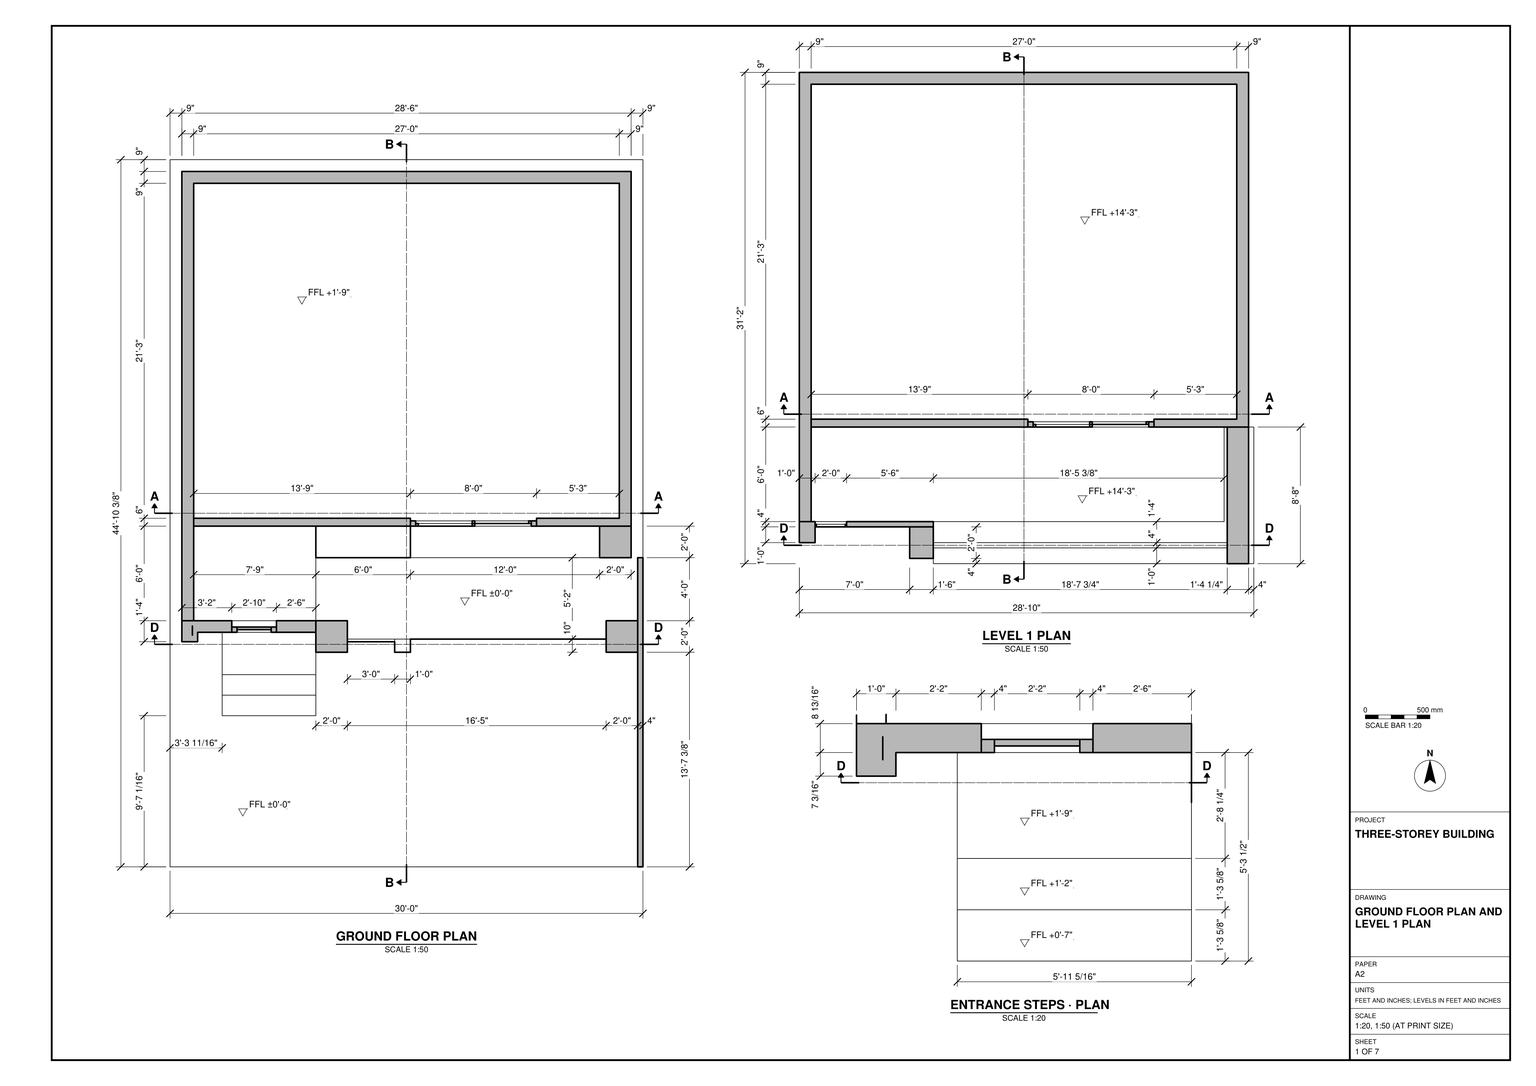
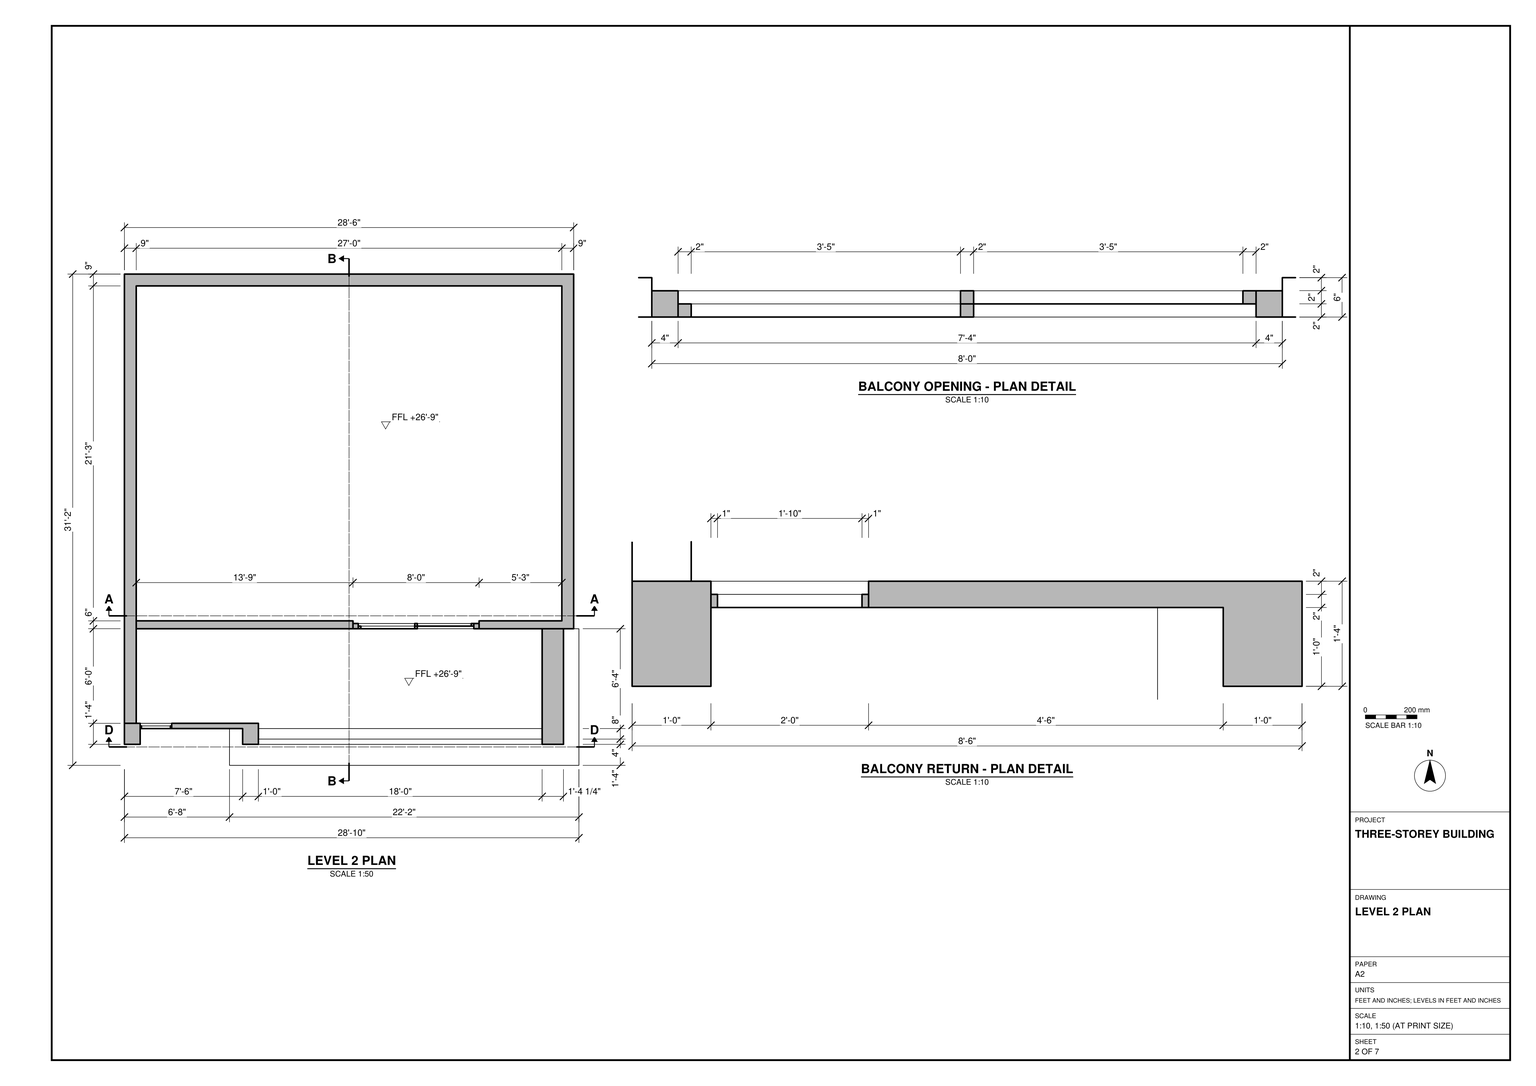
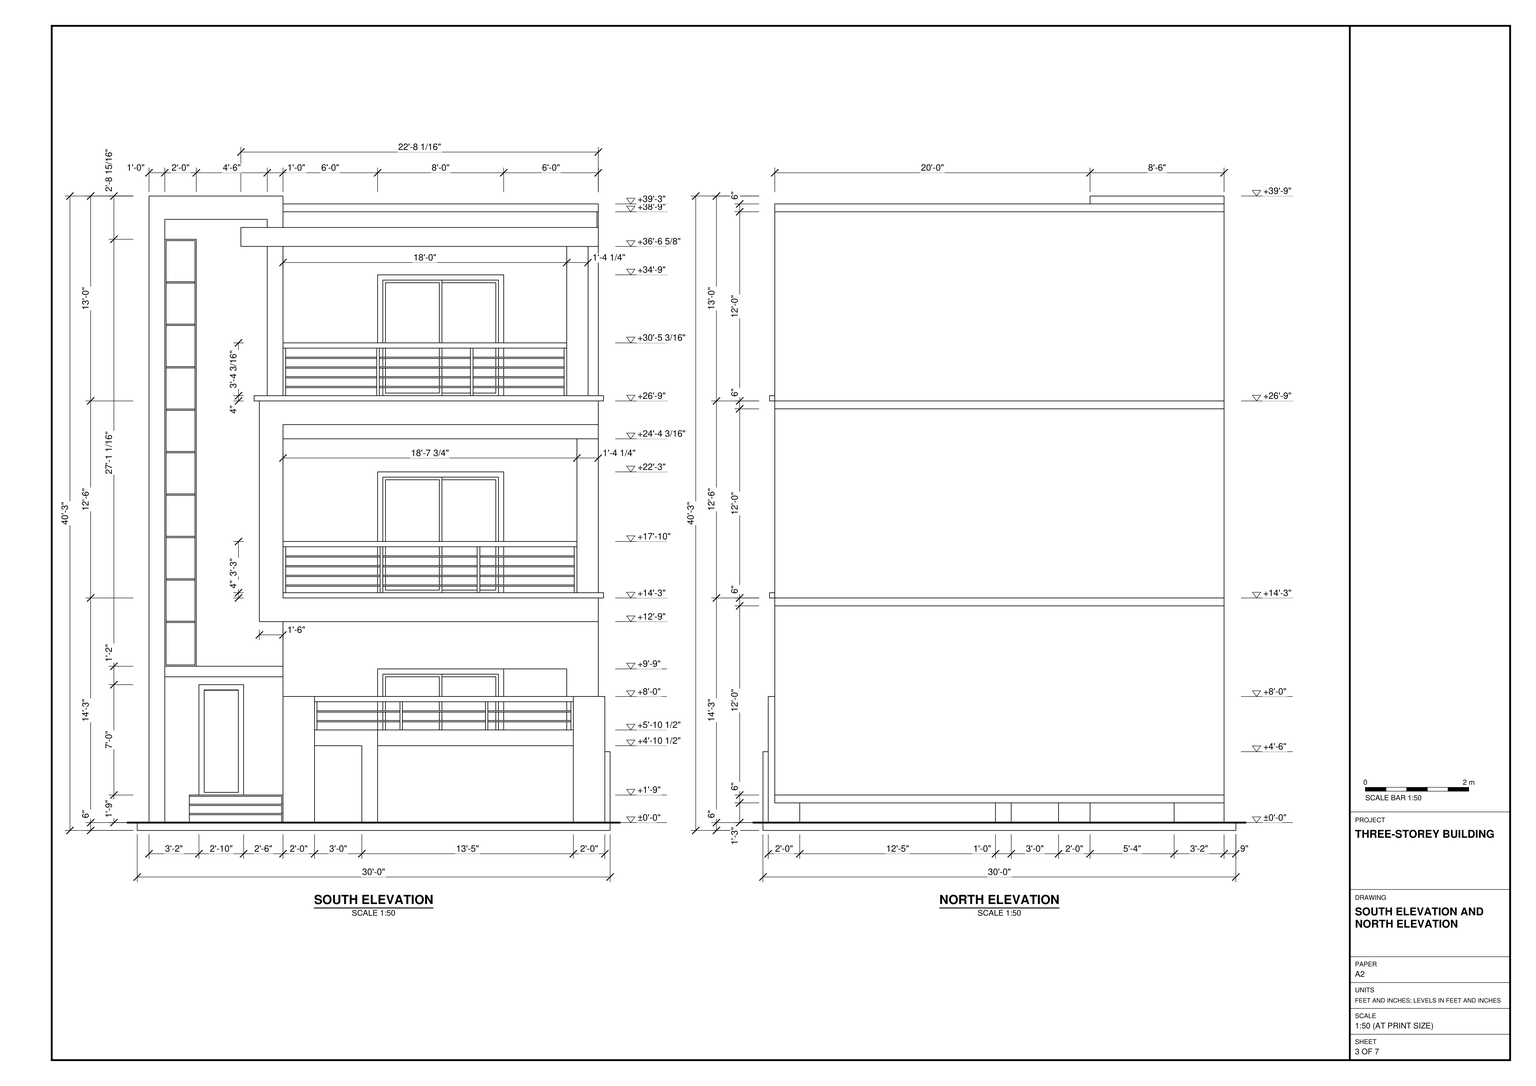
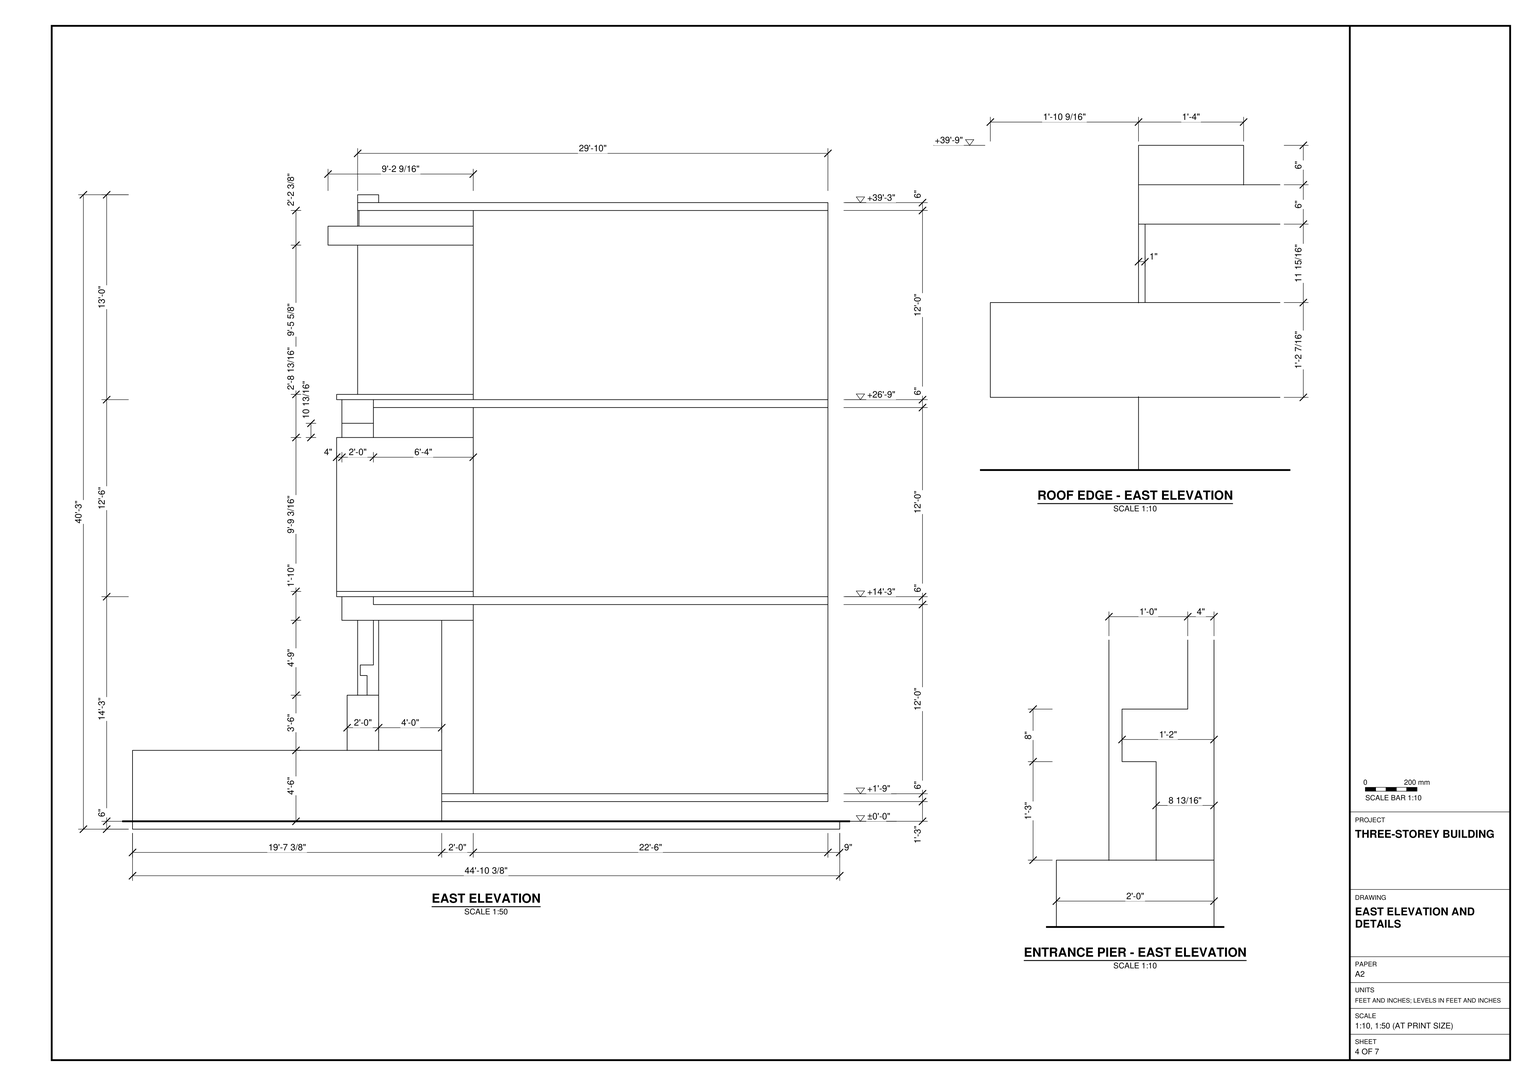
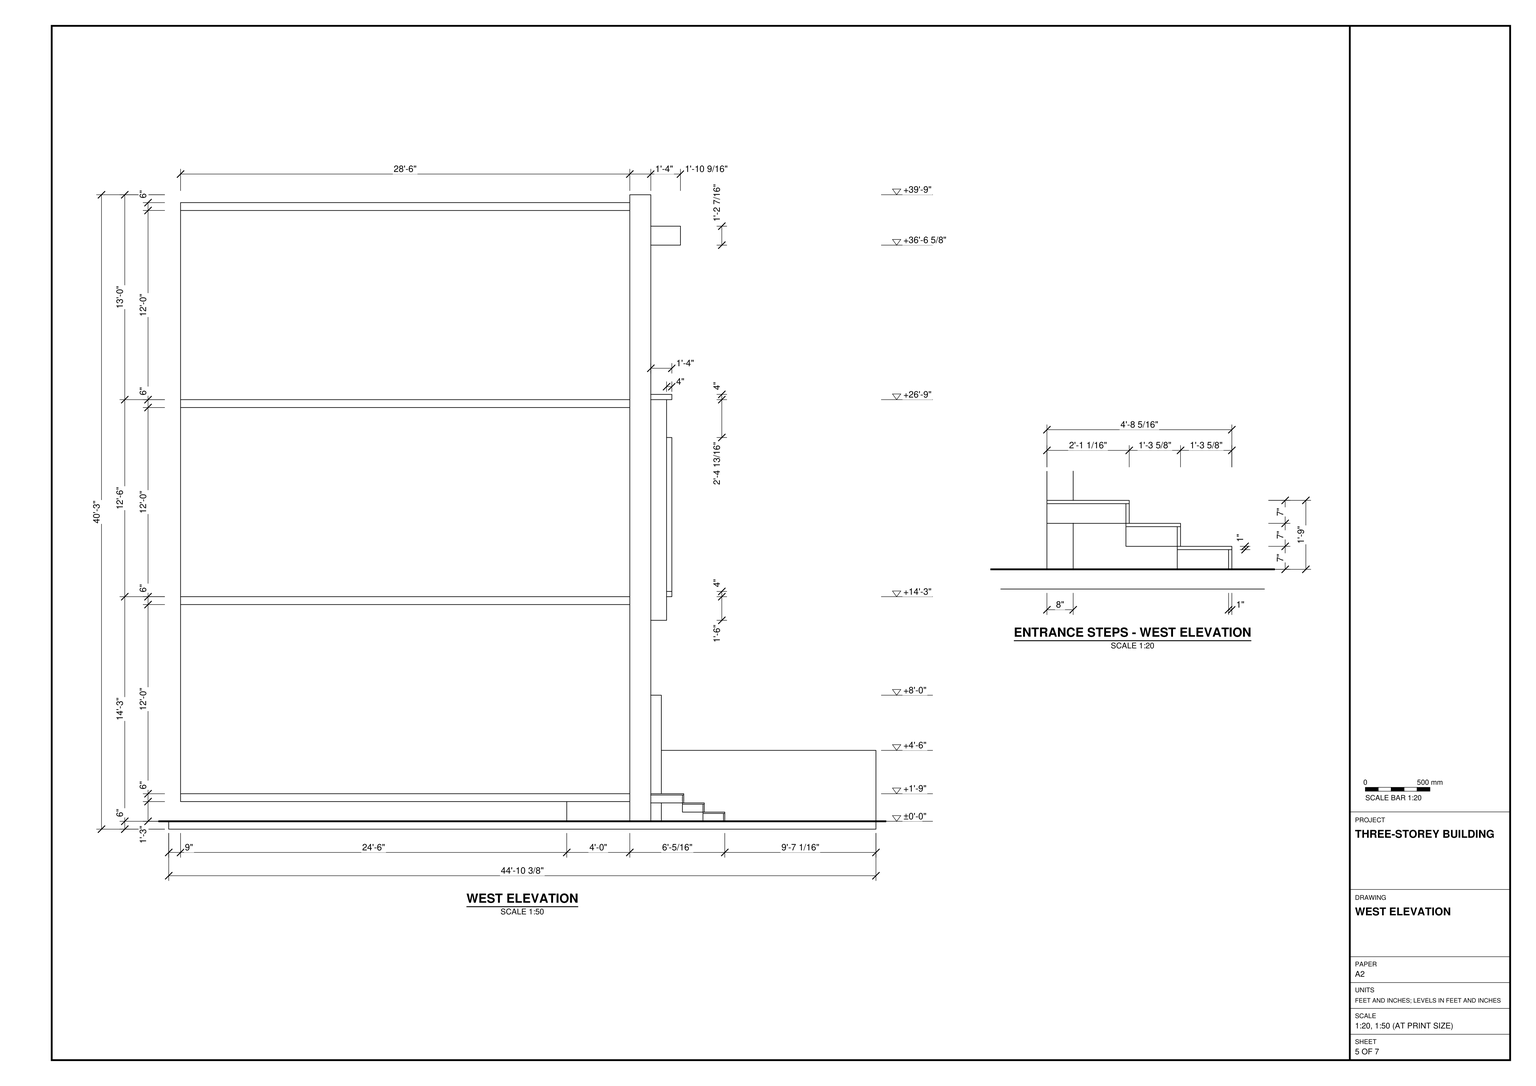
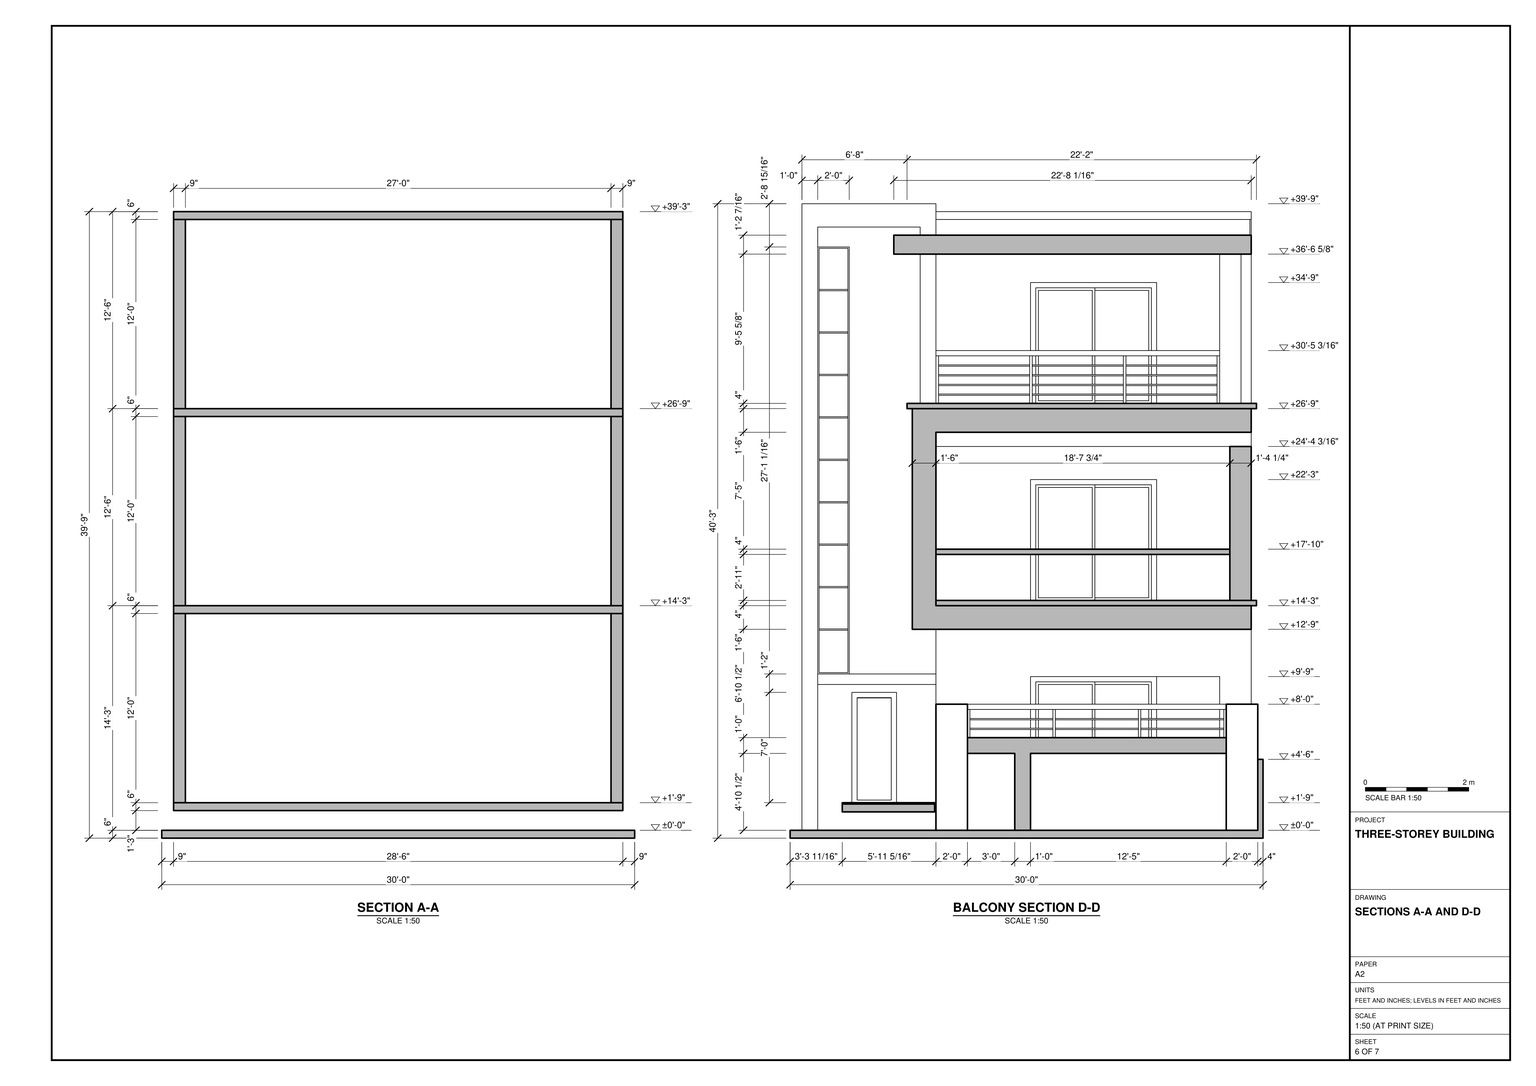
Build the three-storey building shown in task_files/diagram_01.pdf in SketchUp. Work in feet and inches. Include the base and front approach in the overall dimensions of 30'-0" wide, 44'-10 3/8" deep and 40'-3" high. Use ±0'-0" as the ground datum, with Level 1 at +14'-3" and Level 2 at +26'-9". The enclosed ground floor is raised above the approach to +1'-9".

Lay out the rectangular enclosed space on each floor with 9" side and rear walls and a 6" wall facing the front porch or balcony. Model the floor slabs, the entrance steps and landing on the left of the south elevation, and the screened porch beside them. Align the paired framed openings vertically behind the porch and balconies. Follow the separate upper-floor plans for the balcony slab edges, supports and short wall returns rather than copying one balcony unchanged. Include the horizontal railings, the tall narrow panel strip above the entrance, and the projecting band at the flat roof. Keep the rear elevation plain as drawn.

Keep walls, slabs and roof separate as groups or components, and do the same for each furniture or joinery piece shown. Use components for repeated parts. Any decor or loose items shown may use suitable library components. Save one SketchUp model as output_files/three_storey_building_with_stacked_front_balconies.skp.

# SketchUp Ruby script. Lengths in inches.
U = 1.inch
M = Sketchup.active_model
def pt(a) = Geom::Point3d.new(a.map { |v| v * U })
def face(e, loops, mat)
  f = e.add_face(loops[0].map { |a| pt(a) })
  loops[1..].each { |l| e.add_face(l.map { |a| pt(a) }).erase! }
  f.material = f.back_material = mat if mat
  f
end
# faces: each face lists its corners as indices into pts; further lists are holes
def faces(e, pts, list, mat = nil) = list.each { |f| face(e, (f[0].is_a?(Array) ? f : [f]).map { |l| l.map { |i| pts[i] } }, mat) }
# xy, xz, yz: faces in a plane at the given z, y or x. An outline is a flat list of corners, or four numbers for a rectangle; further outlines are holes
def ring(l) = l.size == 4 ? [[l[0], l[1]], [l[2], l[1]], [l[2], l[3]], [l[0], l[3]]] : l.each_slice(2).to_a
def flat(e, list, mat, &to3) = list.each { |f| face(e, (f[0].is_a?(Array) ? f : [f]).map { |l| ring(l).map { |u, v| to3.(u, v) } }, mat) }
def xy(e, z, list, mat = nil) = flat(e, list, mat) { |x, y| [x, y, z] }
def xz(e, y, list, mat = nil) = flat(e, list, mat) { |x, z| [x, y, z] }
def yz(e, x, list, mat = nil) = flat(e, list, mat) { |y, z| [x, y, z] }
def lines(e, pts, list) = list.each { |a, b| e.add_line(pt(pts[a]), pt(pts[b])) }
# prism: a flat outline (further loops are holes) pulled along v
def prism(e, loops, v, mat = nil)
  f = face(e, loops, mat); d = Geom::Vector3d.new(v.map { |x| x * U })
  f.pushpull(f.normal.samedirection?(d) ? d.length : -d.length)
end
def box(e, o, s, mat = nil) = prism(e, [[o, [o[0] + s[0], o[1], o[2]], [o[0] + s[0], o[1] + s[1], o[2]], [o[0], o[1] + s[1], o[2]]]], [0, 0, s[2]], mat)
def at(x, y, z, deg = 0) = Geom::Transformation.translation(pt([x, y, z])) * Geom::Transformation.rotation(ORIGIN, Z_AXIS, deg.degrees)
def axes(o, x, y, z) = Geom::Transformation.new([*x, 0, *y, 0, *z, 0, *pt(o).to_a, 1])
def part(name) = M.definitions.add(name)
# library, detail: a bought-in or finely detailed component or shape, given as its bounding box
def library(name, o, s) = part(name).tap { |d| box(d.entities, o, s) }
def detail(e, o, s) = box(e.add_group.entities, o, s)
def put(e, d, t, mat = nil) = e.add_instance(d, t).tap { |i| i.material = mat if mat }
def group(e, t, mat = nil) = e.add_group.tap { |g| g.transformation = t; g.material = mat if mat }.entities
root = M.entities
M.materials.add("[Carpet Berber Pattern Gray]").color = [165, 165, 165]
M.materials.add("[Color K02]").color = [255, 153, 255]
M.materials.add("[Color M05]").color = [114, 114, 114]
M.materials.add("[Color M06]").color = [86, 86, 86]
M.materials.add("[Color M07]").color = [58, 58, 58]
M.materials.add("[Concrete Tile]").color = [163, 163, 163]
M.materials.add("[Fabric Linen]").color = [161, 161, 136]
M.materials.add("[Roofing Slate Tan]").color = [200, 175, 128]
M.materials.add("[Sketchy Siding Scale]").color = [244, 244, 244]
M.materials.add("[Sketchy Stone Ashlar]").color = [168, 168, 168]
M.materials.add("[Slate Light Tile]").color = [54, 54, 54]
M.materials.add("[Translucent Glass Gray]").color = [128, 128, 128]
M.materials["[Translucent Glass Gray]"].alpha = 0.86
M.materials.add("[Translucent Glass Gray]1").color = [33, 33, 33]
M.materials["[Translucent Glass Gray]1"].alpha = 0.5
M.materials.add("[Wood Floor Light]").color = [197, 155, 82]
c1 = part("Group\#10")
g1 = group(c1.entities,at(4,0,4))
xy(g1,0,[[0,0,45,2]])
xy(g1,2,[[2,0,43,2]])
xy(g1,86,[[2,0,43,2]])
xy(g1,88,[[0,0,45,2]])
xz(g1,0,[[[0,0,45,88],[2,2,43,86]]])
xz(g1,0,[[2,2,43,86]],"[Translucent Glass Gray]")
xz(g1,2,[[[0,0,45,88],[2,2,43,86]]])
yz(g1,0,[[0,0,2,88]])
yz(g1,2,[[0,2,2,86]])
yz(g1,43,[[0,2,2,86]])
yz(g1,45,[[0,0,2,88]])
g2 = group(c1.entities,at(47,2,4))
xy(g2,0,[[0,0,45,2]])
xy(g2,2,[[2,0,43,2]])
xy(g2,86,[[2,0,43,2]])
xy(g2,88,[[0,0,45,2]])
xz(g2,0,[[[0,0,45,88],[2,2,43,86]]])
xz(g2,0,[[2,2,43,86]],"[Translucent Glass Gray]")
xz(g2,2,[[[0,0,45,88],[2,2,43,86]]])
yz(g2,0,[[0,0,2,88]])
yz(g2,2,[[0,2,2,86]])
yz(g2,43,[[0,2,2,86]])
yz(g2,45,[[0,0,2,88]])
g3 = group(c1.entities,at(0,0,0))
prism(g3,[[[0,4,96],[96,4,96],[96,4,0],[0,4,0]],[[4,4,4],[92,4,4],[92,4,92],[4,4,92]]],[0,-4,0])
c2 = part("Group\#20")
box(c2.entities,[0,0,0],[24,24,96])
g4 = group(root,at(0,178.375,0))
xy(g4,-6,[[0,-178.375,360,360]])
xy(g4,0,[[0,-178.375,356,-178.375,356,57,360,57,360,360,0,360]],"[Sketchy Stone Ashlar]")
xy(g4,54,[[356,-178.375,360,57]],"[Color M05]")
xz(g4,-178.375,[[0,-6,360,-6,360,54,356,54,356,0,0,0]],"[Color M05]")
xz(g4,57,[[356,0,360,54]])
xz(g4,360,[[0,-6,360,0]])
yz(g4,0,[[-178.375,-6,360,0]])
yz(g4,356,[[-178.375,0,57,54]],"[Color M05]")
yz(g4,360,[[-178.375,-6,360,-6,360,0,57,0,57,54,-178.375,54]],"[Color M05]")
g5 = group(root,at(9,106.75,15))
prism(g5,[[[0,422.625,0],[342,422.625,0],[342,128.625,0],[102,128.625,0],[102,80.625,0],[0,80.625,0]]],[0,0,6])
p = [[333,413.625,6],[9,413.625,6]]
lines(g5,p,[[0,1]])
g6 = group(root,at(9,171.375,21),"[Sketchy Siding Scale]")
xy(g6,-21,[[0,0,0,12,8,12,8,5,12,5,12,0],[8,5,8,12,0,12,0,16,38,16,38,7.1875,12,7.1875,12,5],[38,7.1875,102,16]])
xy(g6,0,[[38,7.1875,72,16]])
xy(g6,84,[[38,7.1875,72,16]])
xy(g6,90,[[8,2,12,5]])
xy(g6,90,[[12,2,102,7.1875]],"[Color M06]")
xy(g6,98,[[8,2,12,12]])
xy(g6,98,[[12,2,102,2,102,12,36,12,36,16,12,16]],"[Color M06]")
xy(g6,300,[[90,0,102,12]])
xy(g6,423.0625,[[12,12,36,16]])
xy(g6,438.25,[[12,0,90,12]],"[Color M06]")
xy(g6,456,[[0,0,102,16]],"[Color M06]")
xz(g6,0,[[0,-21,12,-21,12,438.25,90,438.25,90,300,102,300,102,456,0,456]],"[Color M06]")
xz(g6,2,[[8,90,12,98]])
xz(g6,2,[[12,90,102,98]],"[Color M06]")
xz(g6,7.1875,[[[12,-21,102,90],[38,0,72,84]]])
xz(g6,12,[[36,98,102,98,102,300,90,300,90,438.25,12,438.25,12,423.0625,36,423.0625]],"[Concrete Tile]")
xz(g6,16,[[[0,-21,0,456,102,456,102,-21,38,-21,38,0,72,0,72,84,38,84,38,-21],[12,98,36,423.0625]]])
yz(g6,0,[[0,-21,16,456]],"[Color M06]")
yz(g6,8,[[5,-21,12,90],[2,90,12,98]])
yz(g6,12,[[0,-21,7.1875,-21,7.1875,90,2,90,2,98,16,98,16,423.0625,12,423.0625,12,438.25,0,438.25]])
yz(g6,36,[[12,98,16,423.0625]])
yz(g6,38,[[7.1875,0,16,84]])
yz(g6,72,[[7.1875,0,16,84]])
yz(g6,90,[[0,300,12,438.25]],"[Color M06]")
yz(g6,102,[[7.1875,-21,16,-21,16,456,0,456,0,300,12,300,12,98,2,98,2,90,7.1875,90]],"[Color M06]")
g7 = group(root,at(93,159.375,153),"[Color M07]")
xy(g7,0,[[0,0,0,24,18,24,18,100,258,100,258,0]])
xy(g7,12,[[18,24,258,100]])
xy(g7,18,[[18,0,258,24]])
xy(g7,150,[[18,0,258,24]])
xy(g7,168,[[0,0,258,24]])
xz(g7,0,[[0,0,258,0,258,18,18,18,18,150,258,150,258,168,0,168]])
xz(g7,24,[[0,0,0,168,258,168,258,150,18,150,18,18,258,18,258,12,18,12,18,0]])
xz(g7,100,[[18,0,258,12]])
yz(g7,0,[[0,0,24,168]])
yz(g7,18,[[24,0,100,12],[0,18,24,150]])
yz(g7,258,[[0,0,100,0,100,12,24,12,24,18,0,18],[0,150,24,168]])
g8 = group(root,at(9,187.375,21))
xy(g8,0,[[0,0,0,342,342,342,342,72,270,72,270,78,333,78,333,333,9,333,9,0],[9,72,174,78]])
xy(g8,96,[[174,72,270,78]])
xy(g8,144,[[[0,0,9,0,9,72,342,72,342,342,0,342],[9,78,333,333]]])
xz(g8,0,[[0,0,9,144]])
xz(g8,72,[[9,0,174,0,174,96,270,96,270,0,342,0,342,144,9,144]],"[Roofing Slate Tan]")
xz(g8,78,[[9,0,9,144,333,144,333,0,270,0,270,96,174,96,174,0]])
xz(g8,333,[[9,0,333,144]])
xz(g8,342,[[0,0,342,144]])
yz(g8,0,[[0,0,342,144]])
yz(g8,9,[[0,0,72,144],[72,0,78,144],[78,0,333,144]])
yz(g8,174,[[72,0,78,96]])
yz(g8,270,[[72,0,78,96]])
yz(g8,333,[[78,0,333,144]])
yz(g8,342,[[72,0,342,144]])
put(root,c1,at(183,259.375,21),"[Slate Light Tile]")
g9 = group(root,at(9,187.375,171))
xy(g9,0,[[0,0,0,342,342,342,342,72,270,72,270,78,333,78,333,333,9,333,9,0],[9,72,174,78]])
xy(g9,96,[[174,72,270,78]])
xy(g9,144,[[[0,0,9,0,9,72,342,72,342,342,0,342],[9,78,333,333]]])
xz(g9,0,[[0,0,9,144]])
xz(g9,72,[[9,0,174,0,174,96,270,96,270,0,342,0,342,144,9,144]],"[Wood Floor Light]")
xz(g9,78,[[9,0,9,144,333,144,333,0,270,0,270,96,174,96,174,0]])
xz(g9,333,[[9,0,333,144]])
xz(g9,342,[[0,0,342,144]])
yz(g9,0,[[0,0,342,144]])
yz(g9,9,[[0,0,72,144],[72,0,78,144],[78,0,333,144]])
yz(g9,174,[[72,0,78,96]])
yz(g9,270,[[72,0,78,96]])
yz(g9,333,[[78,0,333,144]])
yz(g9,342,[[72,0,342,144]])
g10 = group(root,at(9,183.375,315))
prism(g10,[[[0,346,0],[342,346,0],[342,0,0],[102,0,0],[102,4,0],[0,4,0]]],[0,0,6])
put(root,c1,at(183,259.375,171),"[Slate Light Tile]")
g11 = group(root,at(9,187.375,321))
xy(g11,0,[[0,0,0,342,342,342,342,72,270,72,270,78,333,78,333,333,9,333,9,0],[9,72,174,78]])
xy(g11,96,[[174,72,270,78]])
xy(g11,144,[[[0,0,9,0,9,72,342,72,342,342,0,342],[9,78,333,333]]])
xz(g11,0,[[0,0,9,144]])
xz(g11,72,[[9,0,174,0,174,96,270,96,270,0,342,0,342,144,9,144]],"[Fabric Linen]")
xz(g11,78,[[9,0,9,144,333,144,333,0,270,0,270,96,174,96,174,0]])
xz(g11,333,[[9,0,333,144]])
xz(g11,342,[[0,0,342,144]])
yz(g11,0,[[0,0,342,144]])
yz(g11,9,[[0,0,72,144],[72,0,78,144],[78,0,333,144]])
yz(g11,174,[[72,0,78,96]])
yz(g11,270,[[72,0,78,96]])
yz(g11,333,[[78,0,333,144]])
yz(g11,342,[[72,0,342,144]])
g12 = group(root,at(9,183.375,465),"[Color M06]")
prism(g12,[[[0,346,0],[342,346,0],[342,-12,0],[102,-12,0],[102,4,0],[0,4,0]]],[0,0,6])
put(root,c1,at(183,259.375,321),"[Slate Light Tile]")
g13 = group(root,at(111,235.375,21),"[Carpet Berber Pattern Gray]")
prism(g13,[[[216,24,96],[72,24,96],[72,24,0],[0,24,0],[0,24,132],[240,24,132],[240,24,0],[216,24,0]]],[0,-24,0])
g14 = group(root,at(9,183.375,165))
prism(g14,[[[0,346,0],[342,346,0],[342,0,0],[102,0,0],[102,4,0],[0,4,0]]],[0,0,6])
g15 = group(root,at(111,155.375,171),"[Color M07]")
prism(g15,[[[244,104,0],[244,0,0],[0,0,0],[0,32,0],[221.375,32,0],[221.375,104,0]]],[0,0,4])
g16 = group(root,at(111,183.375,292.1875),"[Sketchy Siding Scale]")
xy(g16,0,[[0,0,240,76]],"[Wood Floor Light]")
xy(g16,22.8125,[[0,0,240,76]])
xz(g16,0,[[0,0,240,22.8125]])
xz(g16,76,[[0,0,240,22.8125]])
yz(g16,0,[[0,0,76,22.8125]])
yz(g16,240,[[0,0,76,22.8125]])
g17 = group(root,at(334.75,155.375,175),"[Color M06]")
box(g17,[0,0,0],[16.25,104,117.1875])
g18 = group(root,at(93,159.375,321),"[Color M07]")
prism(g18,[[[-4,24,0],[6,24,0],[6,12,0],[18,12,0],[18,24,0],[234,24,0],[234,100,0],[262,100,0],[262,-4,0],[-4,-4,0]]],[0,0,4])
g19 = group(root,at(327,155.375,325),"[Color M06]")
box(g19,[0,16,0],[16.25,88,117.1875])
g20 = group(root,at(111,167.375,173),"[Slate Light Tile]")
xy(g20,0,[[0,0,2.07,2],[73.89,0,75.96,2],[147.79,0,149.86,2],[221.68,0,223.75,2]])
xy(g20,6.9,[[0,1,73.89,2],[73.89,1,147.79,2],[147.79,1,221.68,2],[221.68,1,223.75,2]])
xy(g20,7.9,[[0,1,73.89,2],[73.89,1,147.79,2],[147.79,1,221.68,2],[221.68,1,223.75,2]])
xy(g20,14.3,[[0,1,73.89,2],[73.89,1,147.79,2],[147.79,1,221.68,2],[221.68,1,223.75,2]])
xy(g20,15.3,[[0,1,73.89,2],[73.89,1,147.79,2],[147.79,1,221.68,2],[221.68,1,223.75,2]])
xy(g20,21.7,[[0,1,73.89,2],[73.89,1,147.79,2],[147.79,1,221.68,2],[221.68,1,223.75,2]])
xy(g20,22.7,[[0,1,73.89,2],[73.89,1,147.79,2],[147.79,1,221.68,2],[221.68,1,223.75,2]])
xy(g20,29.1,[[0,1,73.89,2],[73.89,1,147.79,2],[147.79,1,221.68,2],[221.68,1,223.75,2]])
xy(g20,30.1,[[0,1,73.89,2],[73.89,1,147.79,2],[147.79,1,221.68,2],[221.68,1,223.75,2]])
xy(g20,37,[[2.07,0,2.07,2,0,2,0,4,223.75,4,223.75,2,221.68,2,221.68,0,149.86,0,149.86,2,147.79,2,147.79,0,75.96,0,75.96,2,73.89,2,73.89,0],[73.89,0,75.96,2],[147.79,0,149.86,2],[221.68,0,223.75,2]])
xy(g20,41,[[0,0,223.75,4]])
xz(g20,0,[[0,0,2.07,37],[73.89,0,75.96,37],[147.79,0,149.86,37],[221.68,0,223.75,37],[0,37,223.75,41]])
xz(g20,1,[[0,6.9,73.89,7.9],[73.89,6.9,147.79,7.9],[147.79,6.9,221.68,7.9],[221.68,6.9,223.75,7.9],[0,14.3,73.89,15.3],
  [73.89,14.3,147.79,15.3],[147.79,14.3,221.68,15.3],[221.68,14.3,223.75,15.3],[0,21.7,73.89,22.7],[73.89,21.7,147.79,22.7],
  [147.79,21.7,221.68,22.7],[221.68,21.7,223.75,22.7],[0,29.1,73.89,30.1],[73.89,29.1,147.79,30.1],[147.79,29.1,221.68,30.1],
  [221.68,29.1,223.75,30.1]])
xz(g20,2,[[0,0,2.07,6.9],[73.89,0,75.96,6.9],[147.79,0,149.86,6.9],[221.68,0,223.75,6.9],[0,6.9,2.07,7.9],
  [2.07,6.9,73.89,7.9],[73.89,6.9,75.96,7.9],[75.96,6.9,147.79,7.9],[147.79,6.9,149.86,7.9],[149.86,6.9,221.68,7.9],
  [221.68,6.9,223.75,7.9],[0,7.9,2.07,14.3],[73.89,7.9,75.96,14.3],[147.79,7.9,149.86,14.3],[221.68,7.9,223.75,14.3],
  [0,14.3,2.07,15.3],[2.07,14.3,73.89,15.3],[73.89,14.3,75.96,15.3],[75.96,14.3,147.79,15.3],[147.79,14.3,149.86,15.3],
  [149.86,14.3,221.68,15.3],[221.68,14.3,223.75,15.3],[0,15.3,2.07,21.7],[73.89,15.3,75.96,21.7],[147.79,15.3,149.86,21.7],
  [221.68,15.3,223.75,21.7],[0,21.7,2.07,22.7],[2.07,21.7,73.89,22.7],[73.89,21.7,75.96,22.7],[75.96,21.7,147.79,22.7],
  [147.79,21.7,149.86,22.7],[149.86,21.7,221.68,22.7],[221.68,21.7,223.75,22.7],[0,22.7,2.07,29.1],[73.89,22.7,75.96,29.1],
  [147.79,22.7,149.86,29.1],[221.68,22.7,223.75,29.1],[0,29.1,2.07,30.1],[2.07,29.1,73.89,30.1],[73.89,29.1,75.96,30.1],
  [75.96,29.1,147.79,30.1],[147.79,29.1,149.86,30.1],[149.86,29.1,221.68,30.1],[221.68,29.1,223.75,30.1],[0,30.1,2.07,37],
  [73.89,30.1,75.96,37],[147.79,30.1,149.86,37],[221.68,30.1,223.75,37]])
xz(g20,4,[[0,37,223.75,41]])
yz(g20,0,[[0,0,0,37,2,37,2,30.1,1,30.1,1,29.1,2,29.1,2,22.7,1,22.7,1,21.7,2,21.7,2,15.3,1,15.3,1,14.3,2,14.3,2,7.9,1,7.9,1,6.9,2,6.9,2,0],[1,6.9,2,7.9],[1,14.3,2,15.3],[1,21.7,2,22.7],[1,29.1,2,30.1],
  [0,37,4,41]])
yz(g20,2.07,[[0,0,2,37]])
yz(g20,73.89,[[0,0,0,37,2,37,2,30.1,1,30.1,1,29.1,2,29.1,2,22.7,1,22.7,1,21.7,2,21.7,2,15.3,1,15.3,1,14.3,2,14.3,2,7.9,1,7.9,1,6.9,2,6.9,2,0],[1,6.9,2,7.9],[1,14.3,2,15.3],[1,21.7,2,22.7],[1,29.1,2,30.1]])
yz(g20,75.96,[[0,0,2,37]])
yz(g20,147.79,[[0,0,0,37,2,37,2,30.1,1,30.1,1,29.1,2,29.1,2,22.7,1,22.7,1,21.7,2,21.7,2,15.3,1,15.3,1,14.3,2,14.3,2,7.9,1,7.9,1,6.9,2,6.9,2,0],[1,6.9,2,7.9],[1,14.3,2,15.3],[1,21.7,2,22.7],[1,29.1,2,30.1]])
yz(g20,149.86,[[0,0,2,37]])
yz(g20,221.68,[[0,0,0,37,2,37,2,30.1,1,30.1,1,29.1,2,29.1,2,22.7,1,22.7,1,21.7,2,21.7,2,15.3,1,15.3,1,14.3,2,14.3,2,7.9,1,7.9,1,6.9,2,6.9,2,0],[1,6.9,2,7.9],[1,14.3,2,15.3],[1,21.7,2,22.7],[1,29.1,2,30.1]])
yz(g20,223.75,[[0,0,2,0,2,6.9,1,6.9,1,7.9,2,7.9,2,14.3,1,14.3,1,15.3,2,15.3,2,21.7,1,21.7,1,22.7,2,22.7,2,29.1,1,29.1,1,30.1,2,30.1,2,37,0,37],[1,6.9,2,7.9],[1,14.3,2,15.3],[1,21.7,2,22.7],[1,29.1,2,30.1],
  [0,37,4,41]])
g21 = group(root,at(111,171.375,324.22),"[Slate Light Tile]")
xy(g21,0,[[0,0,2,2],[71.33,0,73.33,2],[142.67,0,144.67,2],[214,0,216,2]])
xy(g21,6.9,[[0,1,71.33,2],[71.33,1,142.67,2],[142.67,1,214,2],[214,1,216,2]])
xy(g21,7.9,[[0,1,71.33,2],[71.33,1,142.67,2],[142.67,1,214,2],[214,1,216,2]])
xy(g21,14.3,[[0,1,71.33,2],[71.33,1,142.67,2],[142.67,1,214,2],[214,1,216,2]])
xy(g21,15.3,[[0,1,71.33,2],[71.33,1,142.67,2],[142.67,1,214,2],[214,1,216,2]])
xy(g21,21.7,[[0,1,71.33,2],[71.33,1,142.67,2],[142.67,1,214,2],[214,1,216,2]])
xy(g21,22.7,[[0,1,71.33,2],[71.33,1,142.67,2],[142.67,1,214,2],[214,1,216,2]])
xy(g21,29.1,[[0,1,71.33,2],[71.33,1,142.67,2],[142.67,1,214,2],[214,1,216,2]])
xy(g21,30.1,[[0,1,71.33,2],[71.33,1,142.67,2],[142.67,1,214,2],[214,1,216,2]])
xy(g21,37,[[2,0,2,2,0,2,0,4,216,4,216,2,214,2,214,0,144.67,0,144.67,2,142.67,2,142.67,0,73.33,0,73.33,2,71.33,2,71.33,0],[71.33,0,73.33,2],[142.67,0,144.67,2],[214,0,216,2]])
xy(g21,41,[[0,0,216,4]])
xz(g21,0,[[0,0,2,37],[71.33,0,73.33,37],[142.67,0,144.67,37],[214,0,216,37],[0,37,216,41]])
xz(g21,1,[[0,6.9,71.33,7.9],[71.33,6.9,142.67,7.9],[142.67,6.9,214,7.9],[214,6.9,216,7.9],[0,14.3,71.33,15.3],
  [71.33,14.3,142.67,15.3],[142.67,14.3,214,15.3],[214,14.3,216,15.3],[0,21.7,71.33,22.7],[71.33,21.7,142.67,22.7],
  [142.67,21.7,214,22.7],[214,21.7,216,22.7],[0,29.1,71.33,30.1],[71.33,29.1,142.67,30.1],[142.67,29.1,214,30.1],
  [214,29.1,216,30.1]])
xz(g21,2,[[0,0,2,6.9],[71.33,0,73.33,6.9],[142.67,0,144.67,6.9],[214,0,216,6.9],[0,6.9,2,7.9],
  [2,6.9,71.33,7.9],[71.33,6.9,73.33,7.9],[73.33,6.9,142.67,7.9],[142.67,6.9,144.67,7.9],[144.67,6.9,214,7.9],
  [214,6.9,216,7.9],[0,7.9,2,14.3],[71.33,7.9,73.33,14.3],[142.67,7.9,144.67,14.3],[214,7.9,216,14.3],
  [0,14.3,2,15.3],[2,14.3,71.33,15.3],[71.33,14.3,73.33,15.3],[73.33,14.3,142.67,15.3],[142.67,14.3,144.67,15.3],
  [144.67,14.3,214,15.3],[214,14.3,216,15.3],[0,15.3,2,21.7],[71.33,15.3,73.33,21.7],[142.67,15.3,144.67,21.7],
  [214,15.3,216,21.7],[0,21.7,2,22.7],[2,21.7,71.33,22.7],[71.33,21.7,73.33,22.7],[73.33,21.7,142.67,22.7],
  [142.67,21.7,144.67,22.7],[144.67,21.7,214,22.7],[214,21.7,216,22.7],[0,22.7,2,29.1],[71.33,22.7,73.33,29.1],
  [142.67,22.7,144.67,29.1],[214,22.7,216,29.1],[0,29.1,2,30.1],[2,29.1,71.33,30.1],[71.33,29.1,73.33,30.1],
  [73.33,29.1,142.67,30.1],[142.67,29.1,144.67,30.1],[144.67,29.1,214,30.1],[214,29.1,216,30.1],[0,30.1,2,37],
  [71.33,30.1,73.33,37],[142.67,30.1,144.67,37],[214,30.1,216,37]])
xz(g21,4,[[0,37,216,41]])
yz(g21,0,[[0,0,0,37,2,37,2,30.1,1,30.1,1,29.1,2,29.1,2,22.7,1,22.7,1,21.7,2,21.7,2,15.3,1,15.3,1,14.3,2,14.3,2,7.9,1,7.9,1,6.9,2,6.9,2,0],[1,6.9,2,7.9],[1,14.3,2,15.3],[1,21.7,2,22.7],[1,29.1,2,30.1],
  [0,37,4,41]])
yz(g21,2,[[0,0,2,37]])
yz(g21,71.33,[[0,0,0,37,2,37,2,30.1,1,30.1,1,29.1,2,29.1,2,22.7,1,22.7,1,21.7,2,21.7,2,15.3,1,15.3,1,14.3,2,14.3,2,7.9,1,7.9,1,6.9,2,6.9,2,0],[1,6.9,2,7.9],[1,14.3,2,15.3],[1,21.7,2,22.7],[1,29.1,2,30.1]])
yz(g21,73.33,[[0,0,2,37]])
yz(g21,142.67,[[0,0,0,37,2,37,2,30.1,1,30.1,1,29.1,2,29.1,2,22.7,1,22.7,1,21.7,2,21.7,2,15.3,1,15.3,1,14.3,2,14.3,2,7.9,1,7.9,1,6.9,2,6.9,2,0],[1,6.9,2,7.9],[1,14.3,2,15.3],[1,21.7,2,22.7],[1,29.1,2,30.1]])
yz(g21,144.67,[[0,0,2,37]])
yz(g21,214,[[0,0,0,37,2,37,2,30.1,1,30.1,1,29.1,2,29.1,2,22.7,1,22.7,1,21.7,2,21.7,2,15.3,1,15.3,1,14.3,2,14.3,2,7.9,1,7.9,1,6.9,2,6.9,2,0],[1,6.9,2,7.9],[1,14.3,2,15.3],[1,21.7,2,22.7],[1,29.1,2,30.1]])
yz(g21,216,[[0,0,2,0,2,6.9,1,6.9,1,7.9,2,7.9,2,14.3,1,14.3,1,15.3,2,15.3,2,21.7,1,21.7,1,22.7,2,22.7,2,29.1,1,29.1,1,30.1,2,30.1,2,37,0,37],[1,6.9,2,7.9],[1,14.3,2,15.3],[1,21.7,2,22.7],[1,29.1,2,30.1],
  [0,37,4,41]])
g22 = group(root,at(39.6875,116.0625,0),"[Sketchy Siding Scale]")
xy(g22,0,[[70.3125,-1,71.3125,15.625],[0,0,70.3125,15.625]])
xy(g22,6,[[0,-1,70.3125,0],[0,0,70.3125,15.625]])
xy(g22,7,[[0,-1,71.3125,-1,71.3125,14.625,70.3125,14.625,70.3125,15.625,0,15.625],[70.3125,14.625,71.3125,15.625],[0,15.625,70.3125,31.25],[70.3125,15.625,71.3125,31.25]])
xy(g22,13,[[0,14.625,70.3125,15.625],[0,15.625,70.3125,31.25]])
xy(g22,14,[[0,14.625,71.3125,14.625,71.3125,30.25,70.3125,30.25,70.3125,31.25,0,31.25],[70.3125,30.25,71.3125,31.25],[0,31.25,70.3125,62.5],[70.3125,31.25,71.3125,62.5]])
xy(g22,20,[[0,30.25,70.3125,31.25],[0,31.25,70.3125,62.5]])
xy(g22,21,[[0,30.25,71.3125,62.5]])
xz(g22,-1,[[70.3125,0,71.3125,0,71.3125,7,0,7,0,6,70.3125,6]])
xz(g22,0,[[0,0,70.3125,6]],"[Color M07]")
xz(g22,14.625,[[70.3125,7,71.3125,7,71.3125,14,0,14,0,13,70.3125,13]])
xz(g22,15.625,[[0,0,70.3125,6],[70.3125,0,71.3125,6],[0,6,71.3125,7]])
xz(g22,15.625,[[0,7,70.3125,13]],"[Color M07]")
xz(g22,30.25,[[70.3125,14,71.3125,14,71.3125,21,0,21,0,20,70.3125,20]])
xz(g22,31.25,[[0,7,70.3125,13],[70.3125,7,71.3125,13],[0,13,71.3125,14]])
xz(g22,31.25,[[0,14,70.3125,20]],"[Color M07]")
xz(g22,62.5,[[0,14,70.3125,20],[70.3125,14,71.3125,20],[0,20,71.3125,21]])
yz(g22,0,[[0,0,15.625,6],[-1,6,15.625,7],[15.625,7,31.25,13],[14.625,13,31.25,14],[31.25,14,62.5,20],
  [30.25,20,62.5,21]])
yz(g22,70.3125,[[-1,0,0,6],[0,0,15.625,6],[14.625,7,15.625,13],[15.625,7,31.25,13],[30.25,14,31.25,20],
  [31.25,14,62.5,20]])
yz(g22,71.3125,[[-1,0,15.625,7],[14.625,7,31.25,14],[30.25,14,62.5,21]])
put(root,c2,at(111,163.375,0),"[Color M06]")
put(root,c2,at(332,163.375,0),"[Color M06]")
g23 = group(root,at(135,173.375,70.52),"[Slate Light Tile]")
xy(g23,0,[[0,0,1.82,2],[65.06,0,66.88,2],[130.12,0,131.94,2],[195.18,0,197,2]])
xy(g23,6.18,[[0,1,65.06,2],[65.06,1,130.12,2],[130.12,1,195.18,2]])
xy(g23,7.18,[[0,1,65.06,2],[65.06,1,130.12,2],[130.12,1,195.18,2]])
xy(g23,13.58,[[0,1,65.06,2],[65.06,1,130.12,2],[130.12,1,195.18,2]])
xy(g23,14.58,[[0,1,65.06,2],[65.06,1,130.12,2],[130.12,1,195.18,2]])
xy(g23,21.48,[[1.82,0,1.82,2,0,2,0,4,197,4,197,2,195.18,2,195.18,0,131.94,0,131.94,2,130.12,2,130.12,0,66.88,0,66.88,2,65.06,2,65.06,0],[65.06,0,66.88,2],[130.12,0,131.94,2],[195.18,0,197,2]])
xy(g23,25.48,[[0,0,197,4]])
xz(g23,0,[[0,0,1.82,21.48],[65.06,0,66.88,21.48],[130.12,0,131.94,21.48],[195.18,0,197,21.48],[0,21.48,197,25.48]])
xz(g23,1,[[0,6.18,65.06,7.18],[65.06,6.18,130.12,7.18],[130.12,6.18,195.18,7.18],[0,13.58,65.06,14.58],[65.06,13.58,130.12,14.58],
  [130.12,13.58,195.18,14.58]])
xz(g23,2,[[0,0,1.82,6.18],[65.06,0,66.88,6.18],[130.12,0,131.94,6.18],[195.18,0,197,6.18],[0,6.18,1.82,7.18],
  [1.82,6.18,65.06,7.18],[65.06,6.18,66.88,7.18],[66.88,6.18,130.12,7.18],[130.12,6.18,131.94,7.18],[131.94,6.18,195.18,7.18],
  [195.18,6.18,197,7.18],[0,7.18,1.82,13.58],[65.06,7.18,66.88,13.58],[130.12,7.18,131.94,13.58],[195.18,7.18,197,13.58],
  [0,13.58,1.82,14.58],[1.82,13.58,65.06,14.58],[65.06,13.58,66.88,14.58],[66.88,13.58,130.12,14.58],[130.12,13.58,131.94,14.58],
  [131.94,13.58,195.18,14.58],[195.18,13.58,197,14.58],[0,14.58,1.82,21.48],[65.06,14.58,66.88,21.48],[130.12,14.58,131.94,21.48],
  [195.18,14.58,197,21.48]])
xz(g23,4,[[0,21.48,197,25.48]])
yz(g23,0,[[0,0,0,21.48,2,21.48,2,14.58,1,14.58,1,13.58,2,13.58,2,7.18,1,7.18,1,6.18,2,6.18,2,0],[1,6.18,2,7.18],[1,13.58,2,14.58],[0,21.48,4,25.48]])
yz(g23,1.82,[[0,0,2,21.48]])
yz(g23,65.06,[[0,0,0,21.48,2,21.48,2,14.58,1,14.58,1,13.58,2,13.58,2,7.18,1,7.18,1,6.18,2,6.18,2,0],[1,6.18,2,7.18],[1,13.58,2,14.58]])
yz(g23,66.88,[[0,0,2,21.48]])
yz(g23,130.12,[[0,0,0,21.48,2,21.48,2,14.58,1,14.58,1,13.58,2,13.58,2,7.18,1,7.18,1,6.18,2,6.18,2,0],[1,6.18,2,7.18],[1,13.58,2,14.58]])
yz(g23,131.94,[[0,0,2,21.48]])
yz(g23,195.18,[[0,0,0,21.48,2,21.48,2,14.58,1,14.58,1,13.58,2,13.58,2,7.18,1,7.18,1,6.18,2,6.18,2,0],[1,6.18,2,7.18],[1,13.58,2,14.58]])
yz(g23,197,[[0,0,2,21.48],[0,21.48,4,25.48]])
p = [[195.18,1,13.58],[197,1,13.58],[195.18,1,6.18],[197,1,6.18],[195.18,1,14.58],[197,1,14.58],
  [195.18,1,7.18],[197,1,7.18]]
lines(g23,p,[[0,1],[2,3],[4,5],[6,7]])
g24 = group(root,at(135,173.375,0),"[Sketchy Siding Scale]")
xy(g24,0,[[36,-10,48,0],[0,-2,36,0]])
xy(g24,58.52,[[0,-10,36,-2],[48,-10,197,0]])
xy(g24,70.52,[[0,-10,48,0]])
xy(g24,70.52,[[48,-10,197,0]],"[Color M06]")
xz(g24,-10,[[36,0,48,0,48,70.52,0,70.52,0,58.52,36,58.52]])
xz(g24,-10,[[48,58.52,197,70.52]],"[Color M07]")
xz(g24,-2,[[0,0,36,58.52]],"[Wood Floor Light]")
xz(g24,0,[[48,0,197,58.52]],"[Roofing Slate Tan]")
yz(g24,0,[[-2,0,0,58.52],[-10,58.52,0,70.52]])
yz(g24,36,[[-10,0,-2,58.52]])
yz(g24,48,[[-10,0,0,58.52]])
yz(g24,197,[[-10,58.52,0,70.52]])
g25 = group(root,at(78.93,148.8125,438.625),"[Color M06]")
xy(g25,0,[[0,0,272.07,110.5625]])
xy(g25,14.4375,[[0,0,272.07,0,272.07,23.5625,32.07,23.5625,32.07,27.5625,267.07,27.5625,267.07,110.5625,0,110.5625],[32.07,23.5625,271.07,27.5625],[271.07,23.5625,272.07,27.5625],[267.07,27.5625,271.07,110.5625],[271.07,27.5625,272.07,110.5625]])
xy(g25,26.375,[[32.07,23.5625,271.07,27.5625],[267.07,27.5625,271.07,110.5625]])
xz(g25,0,[[0,0,272.07,14.4375]])
xz(g25,23.5625,[[32.07,14.4375,271.07,26.375]],"[Sketchy Siding Scale]")
xz(g25,27.5625,[[32.07,14.4375,267.07,26.375]])
xz(g25,110.5625,[[0,0,272.07,14.4375],[267.07,14.4375,271.07,26.375]])
yz(g25,0,[[0,0,110.5625,14.4375]])
yz(g25,32.07,[[23.5625,14.4375,27.5625,26.375]])
yz(g25,271.07,[[23.5625,14.4375,110.5625,26.375]],"[Sketchy Siding Scale]")
yz(g25,272.07,[[0,0,110.5625,14.4375]])
g26 = group(root,at(47,178.5625,21))
xy(g26,0,[[0,0,34,4]])
xy(g26,2,[[4,0,30,2],[4,2,30,4]])
xy(g26,79.75,[[4,2,30,4]])
xy(g26,80,[[4,0,30,4]])
xy(g26,84,[[0,0,34,4]])
xz(g26,0,[[[0,0,34,84],[4,2,30,80]]],"[Wood Floor Light]")
xz(g26,2,[[4,2,30,79.75]],"[Wood Floor Light]")
xz(g26,4,[[[0,0,34,84],[4,2,30,80]],[4,2,30,79.75]])
yz(g26,0,[[0,0,4,84]])
yz(g26,4,[[0,2,2,2,2,79.75,4,79.75,4,80,0,80],[2,2,4,79.75]])
yz(g26,30,[[0,2,0,80,4,80,4,79.75,2,79.75,2,2],[2,2,4,79.75]])
yz(g26,34,[[0,0,4,84]])
g27 = group(root,at(21,183.375,119))
g28 = group(g27,at(0,2,0),"[Slate Light Tile]")
xy(g28,0,[[0,-2,24,0]],"[Slate Light Tile]")
xy(g28,1,[[1,-2,23,0]],"[Slate Light Tile]")
xy(g28,33.31,[[1,-2,23,0]])
xy(g28,34.31,[[1,-2,23,0]])
xy(g28,65.61,[[1,-2,23,0]])
xy(g28,66.61,[[1,-2,23,0]])
xy(g28,97.92,[[1,-2,23,0]])
xy(g28,98.92,[[1,-2,23,0]])
xy(g28,130.22,[[1,-2,23,0]])
xy(g28,131.23,[[1,-2,23,0]])
xy(g28,162.53,[[1,-2,23,0]])
xy(g28,163.53,[[1,-2,23,0]])
xy(g28,194.84,[[1,-2,23,0]])
xy(g28,195.84,[[1,-2,23,0]])
xy(g28,227.14,[[1,-2,23,0]])
xy(g28,228.14,[[1,-2,23,0]])
xy(g28,259.45,[[1,-2,23,0]])
xy(g28,260.45,[[1,-2,23,0]])
xy(g28,291.76,[[1,-2,23,0]])
xy(g28,292.76,[[1,-2,23,0]])
xy(g28,324.0625,[[1,-2,23,0]],"[Slate Light Tile]")
xy(g28,325.0625,[[0,-2,24,0]],"[Slate Light Tile]")
xz(g28,-2,[[1,33.31,23,34.31],[1,65.61,23,66.61],[1,97.92,23,98.92],[1,130.22,23,131.23],[1,162.53,23,163.53],
  [1,194.84,23,195.84],[1,227.14,23,228.14],[1,259.45,23,260.45],[1,291.76,23,292.76]])
xz(g28,-2,[[[0,0,24,325.0625],[1,1,23,324.0625]]],"[Slate Light Tile]")
xz(g28,0,[[1,33.31,23,34.31],[1,65.61,23,66.61],[1,97.92,23,98.92],[1,130.22,23,131.23],[1,162.53,23,163.53],
  [1,194.84,23,195.84],[1,227.14,23,228.14],[1,259.45,23,260.45],[1,291.76,23,292.76]])
xz(g28,0,[[[0,0,24,325.0625],[1,1,23,324.0625]]],"[Color K02]")
yz(g28,0,[[-2,0,0,325.0625]],"[Slate Light Tile]")
yz(g28,1,[[-2,1,0,33.31],[-2,33.31,0,34.31],[-2,34.31,0,65.61],[-2,65.61,0,66.61],[-2,66.61,0,97.92],
  [-2,97.92,0,98.92],[-2,98.92,0,130.22],[-2,130.22,0,131.23],[-2,131.23,0,162.53],[-2,162.53,0,163.53],
  [-2,163.53,0,194.84],[-2,194.84,0,195.84],[-2,195.84,0,227.14],[-2,227.14,0,228.14],[-2,228.14,0,259.45],
  [-2,259.45,0,260.45],[-2,260.45,0,291.76],[-2,291.76,0,292.76],[-2,292.76,0,324.0625]],"[Slate Light Tile]")
yz(g28,23,[[-2,1,0,33.31],[-2,33.31,0,34.31],[-2,34.31,0,65.61],[-2,65.61,0,66.61],[-2,66.61,0,97.92],
  [-2,97.92,0,98.92],[-2,98.92,0,130.22],[-2,130.22,0,131.23],[-2,131.23,0,162.53],[-2,162.53,0,163.53],
  [-2,163.53,0,194.84],[-2,194.84,0,195.84],[-2,195.84,0,227.14],[-2,227.14,0,228.14],[-2,228.14,0,259.45],
  [-2,259.45,0,260.45],[-2,260.45,0,291.76],[-2,291.76,0,292.76],[-2,292.76,0,324.0625]],"[Slate Light Tile]")
yz(g28,24,[[-2,0,0,325.0625]],"[Slate Light Tile]")
g29 = group(g27,at(1,0,1),"[Translucent Glass Gray]1")
xz(g29,0,[[0,0,22,323.0625]])
